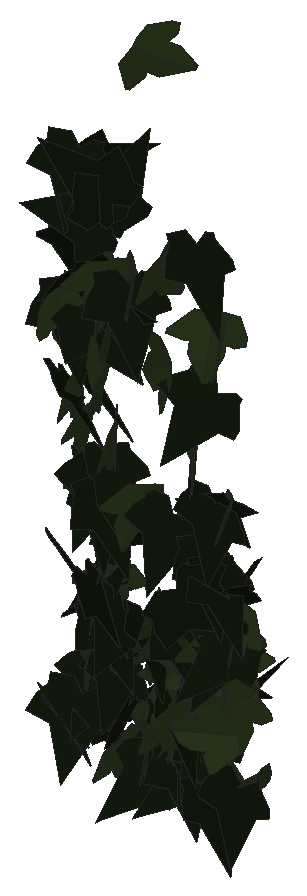
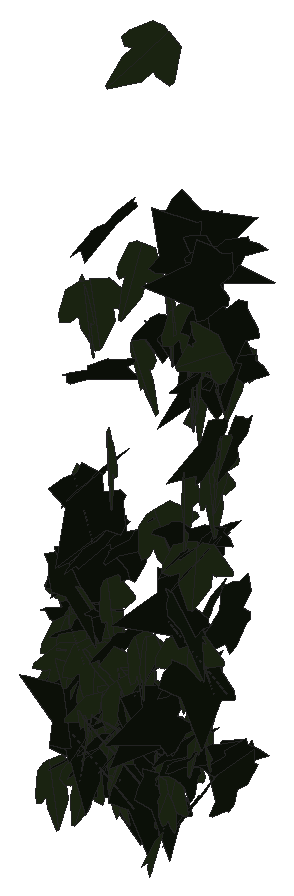
# SketchUp Ruby script. Lengths in inches.
U = 1.inch
M = Sketchup.active_model
def pt(a) = Geom::Point3d.new(a.map { |v| v * U })
def face(e, loops, mat)
  f = e.add_face(loops[0].map { |a| pt(a) })
  loops[1..].each { |l| e.add_face(l.map { |a| pt(a) }).erase! }
  f.material = f.back_material = mat if mat
  f
end
# faces: each face lists its corners as indices into pts; further lists are holes
def faces(e, pts, list, mat = nil) = list.each { |f| face(e, (f[0].is_a?(Array) ? f : [f]).map { |l| l.map { |i| pts[i] } }, mat) }
# xy, xz, yz: faces in a plane at the given z, y or x. An outline is a flat list of corners, or four numbers for a rectangle; further outlines are holes
def ring(l) = l.size == 4 ? [[l[0], l[1]], [l[2], l[1]], [l[2], l[3]], [l[0], l[3]]] : l.each_slice(2).to_a
def flat(e, list, mat, &to3) = list.each { |f| face(e, (f[0].is_a?(Array) ? f : [f]).map { |l| ring(l).map { |u, v| to3.(u, v) } }, mat) }
def xy(e, z, list, mat = nil) = flat(e, list, mat) { |x, y| [x, y, z] }
def xz(e, y, list, mat = nil) = flat(e, list, mat) { |x, z| [x, y, z] }
def yz(e, x, list, mat = nil) = flat(e, list, mat) { |y, z| [x, y, z] }
def lines(e, pts, list) = list.each { |a, b| e.add_line(pt(pts[a]), pt(pts[b])) }
# prism: a flat outline (further loops are holes) pulled along v
def prism(e, loops, v, mat = nil)
  f = face(e, loops, mat); d = Geom::Vector3d.new(v.map { |x| x * U })
  f.pushpull(f.normal.samedirection?(d) ? d.length : -d.length)
end
def box(e, o, s, mat = nil) = prism(e, [[o, [o[0] + s[0], o[1], o[2]], [o[0] + s[0], o[1] + s[1], o[2]], [o[0], o[1] + s[1], o[2]]]], [0, 0, s[2]], mat)
def at(x, y, z, deg = 0) = Geom::Transformation.translation(pt([x, y, z])) * Geom::Transformation.rotation(ORIGIN, Z_AXIS, deg.degrees)
def axes(o, x, y, z) = Geom::Transformation.new([*x, 0, *y, 0, *z, 0, *pt(o).to_a, 1])
def part(name) = M.definitions.add(name)
# library, detail: a bought-in or finely detailed component or shape, given as its bounding box
def library(name, o, s) = part(name).tap { |d| box(d.entities, o, s) }
def detail(e, o, s) = box(e.add_group.entities, o, s)
def put(e, d, t, mat = nil) = e.add_instance(d, t).tap { |i| i.material = mat if mat }
def group(e, t, mat = nil) = e.add_group.tap { |g| g.transformation = t; g.material = mat if mat }.entities
root = M.entities
M.materials.add("efeu1").color = [18, 25, 13]
M.materials.add("efeu2").color = [43, 57, 29]
c1 = part("ivyleaf_9")
p = [[1.54,2.16,1.25],[1.36,2.04,1.19],[-0.21,0.99,0.68],[-0.71,1.11,0.82],[-0.85,0.86,0.67],[-0.8,0.17,0.21],
  [-0.9,-0.01,0.1],[-0.67,-0.16,-0.02],[-0.08,-0.08,-0.05],[-0.03,-0.6,-0.4],[0.65,-0.88,-0.66],[0.83,-0.6,-0.49],
  [1.29,-0.42,-0.43],[1.8125,-0.07,-0.26],[1.21,0.44,0.15]]
faces(c1.entities,p,[[0,1,2,3,4,5,6,7,8,9,10,11,12,13,14]],"efeu1")
c2 = part("ivyleaf_10")
p = [[0,0.5,-0.03],[-0.0625,2.02,-0.43],[-0.19,2.01,-0.46],[-0.54,1.05,-0.29],[-0.52,0.625,-0.18],[-0.83,0.76,-0.28],
  [-1.16,0.64,-0.33],[-1.15,0.33,-0.24],[-0.77,-0.39,0.02],[-0.3,-0.51,0.16],[0.04,-0.48,0.23],[-0.02,2.01,-0.4375],
  [-0.06,2.01,-0.43],[0.04,-0.49,0.23],[0.67,-0.49,0.14],[1.38,0.36,-0.2],[1.375,0.51,-0.24],[0.81,0.65,-0.19],
  [0.62,0.59,-0.15],[0.6,1.09,-0.28],[0.5,1.23,-0.31]]
faces(c2.entities,p,[[0,1,2,3,4,5,6,7,8,9,10],[11,12,0,13,14,15,16,17,18,19,20]],"efeu2")
put(root,c1,axes([509.17,133.7,206.97],[0.30006,-0.58971,0.54178],[0.34425,-0.42738,-0.65585],[0.72302,0.44822,0.08743]))
put(root,c1,axes([509.37,134.36,224.39],[0.30523,0.20575,0.73889],[0.64124,0.39046,-0.36323],[-0.47639,0.65741,-0.01551]))
put(root,c1,axes([509.97,133.21,222.7],[0.59516,0.41705,-0.48408],[-0.49203,-0.15674,-0.70701],[-0.46205,0.70411,0.12934]))
put(root,c1,axes([509.71,133.84,225.28],[-0.40681,-0.68778,-0.14492],[0.13264,0.0911,-0.81291],[0.7462,-0.39116,0.06549]))
put(root,c1,axes([510.12,134.22,210.8],[0.13831,0.78254,-0.04229],[-0.13826,-0.01976,-0.81469],[-0.83491,0.13291,0.12791]))
put(root,c1,axes([510.14,133.07,221.93],[-0.03545,0.82585,0.07801],[0.00772,0.07535,-0.8595],[-0.89556,-0.03204,-0.0105]))
put(root,c2,axes([509.88,133.43,218.09],[0.25204,-0.79084,-0.33038],[0.07858,0.36424,-0.81194],[0.85346,0.20001,0.17232]))
put(root,c1,axes([509.45,133.15,212.74],[0.82453,-0.35959,-0.09504],[-0.08755,0.037,-0.89953],[0.36149,0.82916,-0.00108]))
put(root,c2,axes([509.9,132.72,220.87],[0.24103,0.77907,0.2746],[-0.18177,0.31104,-0.80652],[-0.86961,0.15092,0.24469]))
put(root,c2,axes([509.625,134.47,208.93],[0.28794,-0.50678,0.50152],[0.40194,-0.33423,-0.57928],[0.63973,0.43809,0.13822]))
put(root,c2,axes([510.01,134.57,209.18],[-0.63541,0.50574,0.07927],[-0.10753,0.0007,-0.80411],[-0.5418,-0.59326,0.06663]))
put(root,c2,axes([509.35,134.4,222.03],[0.43699,0.01731,0.69402],[0.69017,0.21554,-0.40879],[-0.20841,0.75006,0.10145]))
put(root,c2,axes([509.89,136.49,206.1875],[-0.21515,0.64912,-0.09122],[0.04438,-0.07912,-0.70596],[-0.70602,-0.20278,-0.01657]))
put(root,c1,axes([509.77,134.73,206.89],[0.43721,-0.54375,-0.30686],[-0.15992,0.2572,-0.70423],[0.64872,0.42987,0.0332]))
put(root,c2,axes([510.15,133.65,217.08],[0.09473,-0.79503,-0.13841],[0.01096,0.13495,-0.83146],[0.87051,0.08482,0.02553]))
put(root,c1,axes([510.03,134.7,208.17],[-0.40846,-0.71559,0.1997],[0.04352,-0.25055,-0.80878],[0.74165,-0.37941,0.15744]))
put(root,c1,axes([509.6,133.21,218.22],[0.60663,-0.5959,0.09251],[0.0633,-0.06699,-0.85164],[0.64761,0.56473,-0.00341]))
put(root,c1,axes([510.07,133.48,207.85],[-0.49623,-0.68415,-0.19503],[0.11448,0.1579,-0.84517],[0.70214,-0.50927,-0.00003]))
put(root,c2,axes([509.77,136.2,207.44],[0.51091,-0.33859,0.39054],[0.44547,-0.039,-0.57698],[0.31583,0.60273,0.18206]))
put(root,c1,axes([509.96,133.42,220.86],[-0.25792,-0.80843,-0.33464],[0.06791,0.32933,-0.84794],[0.87232,-0.26467,-0.03294]))
put(root,c1,axes([510.6,134.34,212.74],[-0.32147,0.67597,0.29907],[-0.10991,0.26934,-0.768],[-0.78571,-0.31425,-0.01493]))
put(root,c2,axes([510.22,135.51,207.3125],[-0.72248,0.16898,-0.00185],[0.0019,-0.00029,-0.71758],[-0.1825,-0.66897,-0.00016]))
put(root,c1,axes([510.61,134.54,212.04],[-0.78522,0.26851,-0.10777],[0.09669,-0.05657,-0.80574],[-0.29542,-0.73222,0.02273]))
put(root,c2,axes([510.36,134.15,214.67],[-0.72543,-0.40772,-0.01228],[0.01042,0.00686,-0.81718],[0.4404,-0.67176,-0.00089]))
put(root,c2,axes([510.125,134.09,211.29],[0.52049,-0.5043,0.40472],[0.31158,-0.26227,-0.72503],[0.61335,0.56118,0.02486]))
put(root,c2,axes([510.47,134.39,211.58],[-0.65783,-0.46086,-0.02161],[0.01749,0.01303,-0.79436],[0.49793,-0.60932,-0.00064]))
put(root,c1,axes([510.65,135.21,207.09],[-0.06571,0.72601,0.0827],[-0.02069,0.07818,-0.75759],[-0.78851,-0.06256,0.01299]))
put(root,c1,axes([509.94,133.76,218.4],[0.68696,-0.514,-0.02809],[-0.00831,0.03344,-0.85022],[0.55583,0.63577,0.02201]))
put(root,c1,axes([510.42,133.87,214.87],[-0.19799,-0.73447,0.25799],[-0.0704,-0.2394,-0.78727],[0.83429,-0.1945,-0.00521]))
put(root,c1,axes([511.375,132.99,223.88],[-0.53644,0.14096,0.7455],[-0.7253,0.17269,-0.55456],[-0.22268,-0.90206,0.01034]))
put(root,c1,axes([510.47,134.82,208.39],[-0.21743,-0.69193,0.18857],[0.02478,-0.19451,-0.74548],[0.77212,-0.18861,0.07702]))
put(root,c2,axes([510.67,134.34,210.46],[0.33386,-0.79636,0.07531],[0.0127,-0.07631,-0.86333],[0.79981,0.33363,-0.01772]))
put(root,c2,axes([510.77,133.375,221.21],[0.53089,-0.6513,-0.35879],[-0.01818,0.42936,-0.80628],[0.74336,0.47563,0.23652]))
put(root,c1,axes([510.33,133.41,220.48],[0.28299,-0.64597,-0.57979],[0.03499,0.61782,-0.67126],[0.8673,0.18585,0.21626]))
put(root,c1,axes([510.45,133.89,214.34],[0.10071,-0.79279,0.17038],[0.01666,-0.16314,-0.83018],[0.87415,0.09445,-0.00381]))
put(root,c1,axes([510.54,134.09,215.48],[-0.29985,-0.61593,-0.42198],[0.33662,0.29496,-0.68746],[0.72195,-0.39334,0.14527]))
put(root,c1,axes([510.56,134,210.58],[0.16223,-0.76049,-0.37401],[-0.08246,0.36483,-0.77759],[0.84346,0.18194,-0.00409]))
put(root,c1,axes([511.51,132.98,224.66],[-0.03605,0.03054,0.93121],[-0.86299,0.35017,-0.04489],[-0.35119,-0.86362,0.01472]))
put(root,c2,axes([510.9375,133.83,216.63],[0.32191,-0.77143,-0.31296],[-0.00307,0.33444,-0.82754],[0.83249,0.29954,0.11796]))
put(root,c1,axes([510.43,134.26,212.94],[0.58962,0.2061,0.56163],[0.51379,0.26172,-0.60405],[-0.35458,0.72194,0.05864]))
put(root,c1,axes([510.68,133.75,214.57],[0.15556,-0.81738,-0.29249],[-0.02353,0.29307,-0.83151],[0.86782,0.15446,0.02989]))
put(root,c1,axes([510.57,134.9,209.47],[0.75664,0.04845,0.26768],[0.27088,0.08753,-0.72715],[-0.08144,0.74122,0.06837]))
put(root,c2,axes([511.21,133.21,222.14],[-0.48414,-0.77953,0.06666],[0.02312,-0.09261,-0.91509],[0.78203,-0.47985,0.06832]))
put(root,c2,axes([511.12,133.4,220.43],[0.48252,-0.75218,-0.18376],[0.01978,0.22842,-0.88306],[0.77405,0.46305,0.13712]))
put(root,c1,axes([510.79,132.92,212.16],[0.59398,-0.59289,-0.24997],[-0.1899,0.16351,-0.83906],[0.61477,0.62335,-0.01766]))
put(root,c2,axes([511.39,132.46,219],[0.04593,0.07079,-0.93217],[-0.14846,0.922,0.0627],[0.92299,0.14478,0.05647]))
put(root,c1,axes([510.51,133.36,220.86],[0.33981,-0.18899,0.82754],[0.70035,-0.44124,-0.38835],[0.47963,0.7782,-0.01923]))
put(root,c1,axes([510.96,134.88,209.35],[0.77907,0.23298,0.06754],[0.06844,0.0151,-0.78836],[-0.25209,0.72413,-0.00529]))
put(root,c1,axes([511.48,133.02,207.01],[0.0419,0.3968,0.84355],[0.13812,0.83244,-0.39844],[-0.92193,0.14275,-0.02135]))
put(root,c1,axes([511.34,133.04,224.11],[-0.37277,-0.23,0.8205],[0.69485,0.43637,0.438],[-0.49326,0.78851,-0.00306]))
put(root,c1,axes([511.36,133.75,210.92],[-0.22158,-0.72927,0.4041],[0.04938,-0.42888,-0.7469],[0.83228,-0.16871,0.1519]))
put(root,c2,axes([511.69,133.27,206.89],[-0.16002,-0.728,-0.40796],[0.11918,0.3912,-0.74484],[0.82596,-0.19749,0.02843]))
put(root,c1,axes([512.24,134.24,206.35],[-0.07186,0.84748,-0.06127],[-0.00384,-0.06181,-0.85047],[-0.84968,-0.07139,0.00902]))
put(root,c2,axes([512.1,133.68,214.97],[-0.2448,-0.80969,0.25482],[-0.01587,-0.26079,-0.84391],[0.84869,-0.23842,0.05772]))
put(root,c2,axes([512.01,134.33,210.89],[0.24217,-0.78972,-0.26626],[0.04113,0.28826,-0.81756],[0.83238,0.21551,0.11786]))
put(root,c2,axes([512.07,133.24,222.27],[0.54846,-0.71148,-0.19551],[0.00298,0.24574,-0.88592],[0.73785,0.52787,0.14891]))
put(root,c1,axes([511.97,133.26,221.88],[-0.11353,-0.86843,-0.27563],[0.04143,0.27255,-0.8758],[0.91018,-0.12073,0.00549]))
put(root,c1,axes([511.83,134.34,210.4],[0.28328,-0.76236,0.28741],[0.09427,-0.27157,-0.81327],[0.80927,0.29849,-0.00587]))
put(root,c2,axes([512.62,133.95,210.55],[0.1227,-0.85447,0.00344],[-0.00255,-0.00384,-0.86323],[0.85447,0.12269,-0.00307]))
put(root,c2,axes([512.79,134.54,209.3],[-0.28056,-0.73476,0.32647],[-0.03521,-0.33421,-0.78245],[0.80325,-0.27129,0.07972]))
put(root,c1,axes([513.02,133.46,206.69],[-0.72944,-0.37271,0.19206],[-0.14891,-0.12998,-0.81781],[0.39195,-0.74301,0.04673]))
put(root,c2,axes([512.76,134.85,206.43],[0.24997,-0.78312,0.17845],[0.02573,-0.17899,-0.82153],[0.80278,0.24958,-0.02924]))
put(root,c2,axes([512.66,134.8,207.25],[-0.39223,0.72193,-0.14794],[0.04853,-0.14192,-0.82123],[-0.73533,-0.39445,0.02471]))
put(root,c1,axes([513.15,134.75,208.18],[-0.83853,0.03192,0.0324],[-0.03954,-0.21612,-0.81051],[-0.02247,-0.81085,0.21731]))
put(root,c1,axes([513.03,134.03,208.35],[0.01861,0.1073,0.85761],[-0.06071,0.85586,-0.10577],[-0.86217,-0.05795,0.02596]))
put(root,c2,axes([512.93,132.83,207.68],[0.45958,-0.61766,-0.38922],[-0.0976,0.40381,-0.75606],[0.72351,0.44682,0.14524]))
put(root,c1,axes([513.2,134.22,206.6875],[-0.07408,0.79468,-0.33772],[0.02852,-0.33652,-0.79812],[-0.86299,-0.07934,0.00262]))
put(root,c2,axes([513.34,133.08,219.96],[0.46365,-0.35778,-0.75299],[-0.50226,0.56781,-0.57906],[0.66539,0.67791,0.0876]))
put(root,c2,axes([513.03,134.4,207.4],[0.09387,-0.83687,-0.10613],[-0.00434,0.1063,-0.84208],[0.84356,0.09367,0.00748]))
put(root,c2,axes([513,134.39,207.53],[0.3414,-0.7606,-0.15971],[0.0461,0.19396,-0.82512],[0.77582,0.32318,0.11932]))
put(root,c1,axes([512.84,134.11,214.37],[-0.19062,-0.82398,0.23187],[-0.0209,-0.23299,-0.84517],[0.85572,-0.18924,0.031]))
put(root,c1,axes([512.65,134.43,207.72],[0.26046,-0.80929,-0.00177],[0.02548,0.01006,-0.84974],[0.80889,0.26028,0.02733]))
put(root,c1,axes([513.76,134.75,207.86],[-0.77817,0.29972,-0.02469],[0.01205,-0.03734,-0.83334],[-0.30049,-0.77767,0.0305]))
put(root,c2,axes([513.375,133.04,223.27],[-0.08355,-0.76376,-0.51858],[0.09533,0.51078,-0.76763],[0.91825,-0.12252,0.03251]))
put(root,c2,axes([513.49,134.22,208.32],[-0.34095,-0.74989,0.18335],[0.03568,-0.21553,-0.81515],[0.77115,-0.32158,0.11878]))
put(root,c1,axes([513.1,134.1,211.02],[0.22187,-0.78855,-0.28779],[-0.06197,0.28147,-0.81902],[0.83714,0.22983,0.01564]))
put(root,c2,axes([513.79,134.64,208.6875],[-0.72792,-0.2466,0.35468],[-0.32674,-0.14031,-0.76813],[0.28258,-0.79748,0.02547]))
put(root,c2,axes([513.2,132.42,230.39],[-0.33079,-0.43591,-0.78512],[0.48528,0.61723,-0.54715],[0.75559,-0.58725,0.0077]))
put(root,c1,axes([513.17,134.63,207.84],[0.05457,-0.81841,-0.20257],[0.02543,0.2045,-0.81935],[0.84272,0.04683,0.03785]))
put(root,c2,axes([513.87,134.45,210.1],[0.66977,0.03856,-0.54108],[-0.54111,-0.01301,-0.67073],[-0.03818,0.86092,0.0141]))
put(root,c2,axes([513.77,134.02,208.36],[-0.47352,-0.62613,0.30879],[-0.07039,-0.32839,-0.77383],[0.69457,-0.46014,0.13209]))
put(root,c2,axes([513.5,134.74,208.91],[0.24577,0.81089,-0.02227],[-0.00625,-0.02138,-0.84732],[-0.81118,0.24585,-0.00022]))
put(root,c1,axes([513.83,134.8125,207.7],[0.05896,0.84178,0.00722],[0.01472,0.0062,-0.84372],[-0.84168,0.05907,-0.01425]))
put(root,c1,axes([514.08,134.89,207.22],[-0.76383,0.32911,0.01305],[-0.01265,0.00361,-0.83171],[-0.32913,-0.76393,0.0017]))
put(root,c1,axes([514.04,134.04,206.72],[-0.72956,-0.32156,0.24439],[-0.20164,-0.14723,-0.79565],[0.34996,-0.75519,0.05105]))
put(root,c1,axes([513.42,134.01,206.86],[-0.05833,-0.80044,-0.22127],[0.08341,0.21505,-0.79991],[0.82626,-0.07821,0.06513]))
put(root,c1,axes([513.29,133.8125,208.45],[0.31873,-0.76764,0.20371],[0.07594,-0.18904,-0.83117],[0.79057,0.32764,-0.00229]))
put(root,c2,axes([513.8,135.03,206.41],[-0.79584,0.22786,-0.01391],[0.01569,0.00429,-0.82777],[-0.22774,-0.79595,-0.00844]))
put(root,c2,axes([513.79,132.85,208.79],[-0.22862,-0.76632,-0.46253],[0.13029,0.44381,-0.7997],[0.88556,-0.26313,-0.00175]))
put(root,c2,axes([513.89,133.75,211.97],[0.13801,-0.84145,-0.17747],[-0.04114,0.17307,-0.8526],[0.85897,0.14348,-0.01232]))
put(root,c2,axes([513.97,134.78,207.88],[-0.55151,0.5725,0.28622],[-0.23041,0.17492,-0.79383],[-0.59715,-0.59623,0.04194]))
put(root,c1,axes([513.57,134.73,207.25],[0.14695,-0.82614,-0.05758],[-0.00956,0.05678,-0.83911],[0.82809,0.14726,0.00053]))
put(root,c2,axes([514,134.37,210.16],[-0.53304,-0.6751,-0.06263],[0.03511,0.05208,-0.86016],[0.67709,-0.53418,-0.0047]))
put(root,c2,axes([513.91,134.53,208.375],[0.18751,-0.82142,0.0966],[0.06809,-0.08338,-0.84121],[0.82428,0.19375,0.04751]))
put(root,c1,axes([513.86,134.79,207.71],[-0.39983,-0.73239,0.12628],[0.02033,-0.15413,-0.82948],[0.74292,-0.38994,0.09067]))
put(root,c2,axes([513.94,133.72,216.93],[0.56408,-0.65991,-0.22821],[0.00151,0.29452,-0.84794],[0.69825,0.53247,0.18619]))
put(root,c2,axes([514.04,134.69,208.86],[0.18669,-0.82918,0.02072],[0.00743,-0.01956,-0.84994],[0.82941,0.18681,0.00295]))
put(root,c2,axes([514.1875,134.26,208.87],[-0.29891,-0.76943,0.24282],[-0.05043,-0.24063,-0.82455],[0.80526,-0.30068,0.0385]))
put(root,c1,axes([514.24,134.55,209.19],[0.50835,0.62386,-0.24385],[-0.26179,-0.09672,-0.79322],[-0.61655,0.55545,0.13575]))
put(root,c1,axes([514.15,133.92,215.35],[0.73572,0.45952,-0.05842],[-0.05087,-0.02883,-0.86743],[-0.46042,0.73747,0.00249]))
put(root,c2,axes([514.5,134.13,210.87],[-0.47854,-0.72045,-0.03433],[0.03678,0.01677,-0.86464],[0.72033,-0.47947,0.02135]))
put(root,c1,axes([514.11,134.89,208.13],[0.1068,0.8293,-0.08372],[0.02763,0.08083,0.83598],[0.83306,-0.109,-0.01699]))
put(root,c1,axes([514.22,133.96,213.74],[0.17197,-0.86263,-0.07627],[-0.01611,0.07456,-0.87961],[0.86585,0.17272,-0.00122]))
put(root,c1,axes([514.88,133.56,212.7],[0.1541,0.79954,-0.30007],[-0.15427,-0.27384,-0.80887],[-0.83995,0.19698,0.09351]))
put(root,c2,axes([514.75,134.28,209.375],[-0.48684,-0.69222,0.04256],[-0.01948,-0.03833,-0.84625],[0.69325,-0.48719,0.0061]))
put(root,c2,axes([515.24,133.38,208.47],[0.10355,0.03091,-0.87008],[-0.8666,-0.08056,-0.106],[-0.08369,0.87251,0.02104]))
put(root,c1,axes([514.63,134.57,210.9],[-0.38627,-0.74123,0.18677],[-0.09124,-0.16306,-0.83582],[0.75893,-0.39686,-0.00543]))
put(root,c1,axes([515.08,134.38,212.7],[-0.43924,0.74291,-0.00144],[0.00308,0.00015,-0.86304],[-0.74291,-0.43925,-0.00273]))
put(root,c2,axes([514.75,134.5,210.74],[-0.46053,-0.7133,-0.13305],[0.09822,0.09486,-0.84849],[0.71892,-0.46989,0.03069]))
put(root,c1,axes([514.8,133.6,219.23],[-0.59463,-0.64309,0.21061],[0.00421,-0.28389,-0.85492],[0.67668,-0.56334,0.1904]))
put(root,c1,axes([514.43,132.49,213.24],[0.08137,-0.18572,-0.95521],[-0.03369,0.95743,-0.18902],[0.97252,0.0487,0.07338]))
put(root,c2,axes([514.93,133.39,221.65],[-0.67393,-0.59584,0.15556],[0.01281,-0.24412,-0.87957],[0.61567,-0.64714,0.18857]))
put(root,c2,axes([514.73,134.6,210.01],[0.26507,0.78867,0.19855],[0.00757,0.20643,-0.83007],[-0.81325,0.25898,0.05699]))
put(root,c2,axes([514.99,135.17,206.07],[-0.04412,-0.82303,-0.06945],[-0.02649,0.07093,-0.82366],[0.82553,-0.04171,-0.03015]))
put(root,c1,axes([514.55,133.17,224.09],[0.21522,-0.88862,-0.13844],[-0.0096,0.14007,-0.91402],[0.89929,0.21417,0.02338]))
put(root,c2,axes([514.94,133.9375,215.36],[0.49701,-0.73368,0.01446],[0.01302,-0.00865,-0.88615],[0.73371,0.49714,0.00592]))
put(root,c1,axes([514.71,133.74,215.53],[-0.01903,-0.8479,0.2664],[0.07396,-0.26705,-0.84468],[0.88568,0.00408,0.07626]))
put(root,c2,axes([515.14,134.15,208.99],[-0.7097,-0.4691,-0.00957],[0.00816,0.005,-0.85073],[0.46913,-0.70975,0.00033]))
put(root,c1,axes([514.64,133.375,206.39],[0.34722,-0.76942,-0.06184],[-0.02177,0.05802,-0.84413],[0.7716,0.34788,0.00401]))
put(root,c2,axes([514.77,134.39,210.7],[0.51009,-0.51401,0.45366],[0.33886,-0.30252,-0.72379],[0.59598,0.61195,0.02325]))
put(root,c1,axes([515.29,134.14,211.15],[-0.73028,-0.41323,0.17129],[-0.08701,-0.19045,-0.8304],[0.43878,-0.72552,0.12042]))
put(root,c1,axes([514.75,133.82,213.41],[0.21836,-0.83992,-0.13754],[0.02667,0.14867,-0.86559],[0.85069,0.21094,0.06244]))
put(root,c2,axes([515.29,133.23,221.45],[0.56434,-0.68067,-0.24253],[-0.08422,0.24368,-0.87985],[0.71766,0.56385,0.08747]))
put(root,c2,axes([515.15,134.25,211.84],[0.85292,-0.14206,-0.02323],[-0.02371,-0.00095,-0.86466],[0.14198,0.85324,-0.00483]))
put(root,c1,axes([514.99,134.48,206.24],[-0.05644,-0.83909,0.0994],[0.00877,-0.1002,-0.84084],[0.84491,-0.05501,0.01537]))
